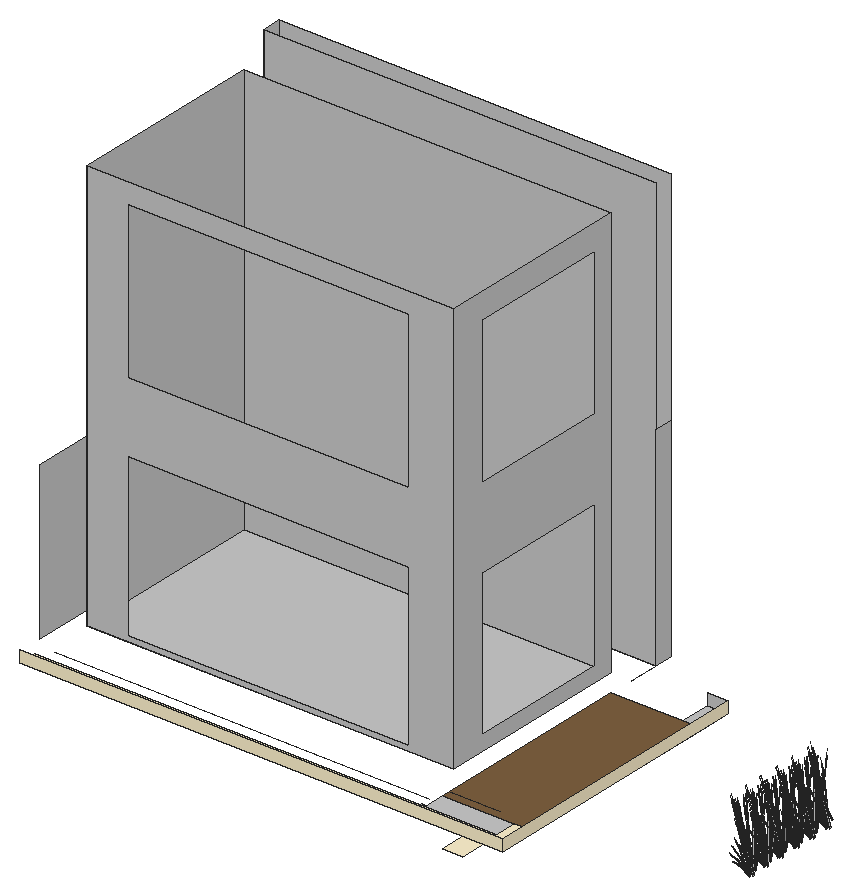
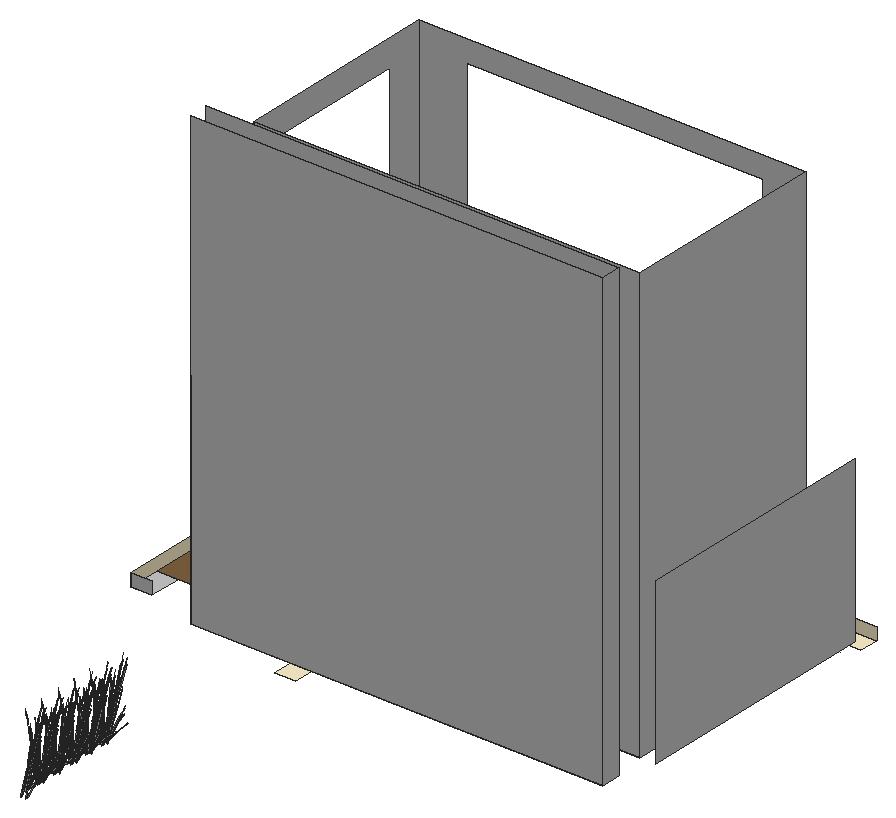
# SketchUp Ruby script. Lengths in inches.
U = 1.inch
M = Sketchup.active_model
def pt(a) = Geom::Point3d.new(a.map { |v| v * U })
def face(e, loops, mat)
  f = e.add_face(loops[0].map { |a| pt(a) })
  loops[1..].each { |l| e.add_face(l.map { |a| pt(a) }).erase! }
  f.material = f.back_material = mat if mat
  f
end
# faces: each face lists its corners as indices into pts; further lists are holes
def faces(e, pts, list, mat = nil) = list.each { |f| face(e, (f[0].is_a?(Array) ? f : [f]).map { |l| l.map { |i| pts[i] } }, mat) }
# xy, xz, yz: faces in a plane at the given z, y or x. An outline is a flat list of corners, or four numbers for a rectangle; further outlines are holes
def ring(l) = l.size == 4 ? [[l[0], l[1]], [l[2], l[1]], [l[2], l[3]], [l[0], l[3]]] : l.each_slice(2).to_a
def flat(e, list, mat, &to3) = list.each { |f| face(e, (f[0].is_a?(Array) ? f : [f]).map { |l| ring(l).map { |u, v| to3.(u, v) } }, mat) }
def xy(e, z, list, mat = nil) = flat(e, list, mat) { |x, y| [x, y, z] }
def xz(e, y, list, mat = nil) = flat(e, list, mat) { |x, z| [x, y, z] }
def yz(e, x, list, mat = nil) = flat(e, list, mat) { |y, z| [x, y, z] }
def lines(e, pts, list) = list.each { |a, b| e.add_line(pt(pts[a]), pt(pts[b])) }
# prism: a flat outline (further loops are holes) pulled along v
def prism(e, loops, v, mat = nil)
  f = face(e, loops, mat); d = Geom::Vector3d.new(v.map { |x| x * U })
  f.pushpull(f.normal.samedirection?(d) ? d.length : -d.length)
end
def box(e, o, s, mat = nil) = prism(e, [[o, [o[0] + s[0], o[1], o[2]], [o[0] + s[0], o[1] + s[1], o[2]], [o[0], o[1] + s[1], o[2]]]], [0, 0, s[2]], mat)
def at(x, y, z, deg = 0) = Geom::Transformation.translation(pt([x, y, z])) * Geom::Transformation.rotation(ORIGIN, Z_AXIS, deg.degrees)
def axes(o, x, y, z) = Geom::Transformation.new([*x, 0, *y, 0, *z, 0, *pt(o).to_a, 1])
def part(name) = M.definitions.add(name)
# library, detail: a bought-in or finely detailed component or shape, given as its bounding box
def library(name, o, s) = part(name).tap { |d| box(d.entities, o, s) }
def detail(e, o, s) = box(e.add_group.entities, o, s)
def put(e, d, t, mat = nil) = e.add_instance(d, t).tap { |i| i.material = mat if mat }
def group(e, t, mat = nil) = e.add_group.tap { |g| g.transformation = t; g.material = mat if mat }.entities
root = M.entities
M.materials.add("D01_Frost_White").color = [255, 242, 206]
M.materials.add("LightPink_Translucent").color = [144, 107, 117]
M.materials["LightPink_Translucent"].alpha = 0.75
M.materials.add("Plywood_01_1K").color = [125, 96, 64]
M.materials.add("[_0053_Ivory_]").color = [200, 200, 200]
c1 = part("blade")
p = [[2.15,0.21,22],[0,0.17,0],[0.09,0.45,0],[2.18,0.31,22],[2.29,0.31,22],[0.38,0.45,0],
  [2.48,0.24,33],[2.49,0.24,33],[2.48,0.22,33]]
faces(c1.entities,p,[[0,1,2,3],[4,5,2,3],[6,3,4,7],[8,0,3,6]])
c2 = part("seeds")
p = [[0.3,-0.1,1.38],[-0.01,-0.03,1.59],[-0.01,-0.03,0.03],[0.14,-0.07,-0.07],[0.29,-0.03,3],[0.15,0.01,3.11]]
faces(c2.entities,p,[[0,1,2,3],[1,0,4,5]],"LightPink_Translucent")
c3 = part("blade with seeds")
put(c3.entities,c1,at(0,0,0))
put(c3.entities,c2,axes([2.4,0.25,30.99],[1.5799,-0.05474,1.17369],[-0.12525,1.92788,0.29478],[-0.07173,-0.02425,1.56792]))
xy(root,81,[[598.7,122.15,610.51,146.15],[598.51,149.15,610.51,170.15],[598.51,173.15,610.51,194.15],[598.51,197.15,610.51,218.15]],"D01_Frost_White")
xy(root,120,[[377.51,83.15,377.51,94.15,653.51,94.15,653.51,107.15,665.51,107.15,665.51,83.15]],"D01_Frost_White")
xy(root,120,[[610.51,107.15,665.51,233.15]],"Plywood_01_1K")
xy(root,120,[[607.51,94.15,607.51,95.51,610.51,95.51,610.51,107.15,653.51,107.15,653.51,94.15],[653.51,233.15,665.51,251.15]],"[_0053_Ivory_]")
xy(root,126,[[386.51,122.15,605.51,239.15],[383.51,257.92,617.51,269.15]],"[_0053_Ivory_]")
xz(root,83.15,[[377.51,120,665.51,127]],"D01_Frost_White")
xz(root,122.15,[[[386.51,126,605.51,372],[410.51,129,578.51,225],[410.51,267,578.51,360]]],"[_0053_Ivory_]")
xz(root,239.15,[[386.51,126,605.51,372]],"[_0053_Ivory_]")
xz(root,251.15,[[653.51,120,665.51,127]],"[_0053_Ivory_]")
xz(root,257.92,[[383.51,126,617.51,384]],"[_0053_Ivory_]")
xz(root,269.15,[[383.51,126,617.51,384]],"[_0053_Ivory_]")
yz(root,377.51,[[98.15,126,239.15,219]],"[_0053_Ivory_]")
yz(root,383.51,[[257.92,126,269.15,384]],"[_0053_Ivory_]")
yz(root,386.51,[[122.15,126,239.15,372]],"[_0053_Ivory_]")
yz(root,605.51,[[[122.15,126,239.15,372],[143.15,270,227.15,357],[143.15,135,227.15,222]]],"[_0053_Ivory_]")
yz(root,617.51,[[257.92,126,269.15,252]],"[_0053_Ivory_]")
yz(root,665.51,[[83.15,120,251.15,127]],"D01_Frost_White")
p = [[617.51,239.15,126],[617.51,257.92,126],[607.51,101.15,120],[383.51,101.15,120],[617.51,104.15,126],[647.51,104.15,126]]
lines(root,p,[[0,1],[2,3],[4,5]])
put(root,c3,axes([672.63,315.29,38.36],[-0.01133,0.07538,1.77383],[-0.55883,0.27355,-0.16761],[-0.16445,-0.13983,0.31391]),"[_0053_Ivory_]")
put(root,c3,axes([672.51,316.63,38.75],[0.67657,-0.16163,0.53763],[0.11742,0.63404,0.4433],[-0.15912,-0.18687,1.11249]),"[_0053_Ivory_]")
put(root,c3,axes([673.27,315.58,38.37],[-0.0929,-0.08817,1.74944],[-0.61994,0.0559,-0.27667],[-0.09894,-0.21089,0.14031]),"[_0053_Ivory_]")
put(root,c3,axes([676.54,254.36,38.37],[-0.09918,0.08165,1.74944],[0.00844,0.59653,-0.27667],[-0.22734,0.07758,0.14031]),"[_0053_Ivory_]")
put(root,c3,axes([676.54,265.51,38.37],[-0.09918,0.08165,1.74944],[0.00844,0.59653,-0.27667],[-0.22734,0.07758,0.14031]),"[_0053_Ivory_]")
put(root,c3,axes([676.54,276.5,38.37],[-0.09918,0.08165,1.74944],[0.00844,0.59653,-0.27667],[-0.22734,0.07758,0.14031]),"[_0053_Ivory_]")
put(root,c3,axes([676.54,288.54,38.37],[-0.09918,0.08165,1.74944],[0.00844,0.59653,-0.27667],[-0.22734,0.07758,0.14031]),"[_0053_Ivory_]")
put(root,c3,axes([676.54,299.91,38.37],[-0.09918,0.08165,1.74944],[0.00844,0.59653,-0.27667],[-0.22734,0.07758,0.14031]),"[_0053_Ivory_]")
put(root,c3,axes([675.4375,254.96,38.36],[0.07751,0.01687,1.77383],[0.23978,0.55562,-0.16761],[-0.15867,0.14583,0.31391]),"[_0053_Ivory_]")
put(root,c3,axes([675.4375,266.11,38.36],[0.07751,0.01687,1.77383],[0.23978,0.55562,-0.16761],[-0.15867,0.14583,0.31391]),"[_0053_Ivory_]")
put(root,c3,axes([675.4375,277.1,38.36],[0.07751,0.01687,1.77383],[0.23978,0.55562,-0.16761],[-0.15867,0.14583,0.31391]),"[_0053_Ivory_]")
put(root,c3,axes([675.4375,289.14,38.36],[0.07751,0.01687,1.77383],[0.23978,0.55562,-0.16761],[-0.15867,0.14583,0.31391]),"[_0053_Ivory_]")
put(root,c3,axes([675.4375,300.51,38.36],[0.07751,0.01687,1.77383],[0.23978,0.55562,-0.16761],[-0.15867,0.14583,0.31391]),"[_0053_Ivory_]")
put(root,c3,axes([677.01,251.875,38.36],[0.04503,0.06276,1.77383],[-0.21706,0.56413,-0.16761],[-0.21983,0.00408,0.31391]),"[_0053_Ivory_]")
put(root,c3,axes([677.01,263.02,38.36],[0.04503,0.06276,1.77383],[-0.21706,0.56413,-0.16761],[-0.21983,0.00408,0.31391]),"[_0053_Ivory_]")
put(root,c3,axes([677.01,274.01,38.36],[0.04503,0.06276,1.77383],[-0.21706,0.56413,-0.16761],[-0.21983,0.00408,0.31391]),"[_0053_Ivory_]")
put(root,c3,axes([677.01,286.06,38.36],[0.04503,0.06276,1.77383],[-0.21706,0.56413,-0.16761],[-0.21983,0.00408,0.31391]),"[_0053_Ivory_]")
put(root,c3,axes([677.01,297.43,38.36],[0.04503,0.06276,1.77383],[-0.21706,0.56413,-0.16761],[-0.21983,0.00408,0.31391]),"[_0053_Ivory_]")
put(root,c3,axes([677.01,309.4,38.36],[0.04503,0.06276,1.77383],[-0.21706,0.56413,-0.16761],[-0.21983,0.00408,0.31391]),"[_0053_Ivory_]")
put(root,c3,axes([677.51,251.5,38.37],[-0.13068,-0.00444,1.74944],[-0.41604,0.44388,-0.27667],[-0.22198,-0.0907,0.14031]),"[_0053_Ivory_]")
put(root,c3,axes([677.51,262.65,38.37],[-0.13068,-0.00444,1.74944],[-0.41604,0.44388,-0.27667],[-0.22198,-0.0907,0.14031]),"[_0053_Ivory_]")
put(root,c3,axes([677.51,273.64,38.37],[-0.13068,-0.00444,1.74944],[-0.41604,0.44388,-0.27667],[-0.22198,-0.0907,0.14031]),"[_0053_Ivory_]")
put(root,c3,axes([677.51,285.68,38.37],[-0.13068,-0.00444,1.74944],[-0.41604,0.44388,-0.27667],[-0.22198,-0.0907,0.14031]),"[_0053_Ivory_]")
put(root,c3,axes([677.51,297.05,38.37],[-0.13068,-0.00444,1.74944],[-0.41604,0.44388,-0.27667],[-0.22198,-0.0907,0.14031]),"[_0053_Ivory_]")
put(root,c3,axes([677.51,309.03,38.37],[-0.13068,-0.00444,1.74944],[-0.41604,0.44388,-0.27667],[-0.22198,-0.0907,0.14031]),"[_0053_Ivory_]")
put(root,c3,axes([676.98,253.95,38.39],[0.17159,-0.57338,0.48003],[0.56413,0.19607,0.3958],[-0.22185,0.03446,0.9933]),"[_0053_Ivory_]")
put(root,c3,axes([676.98,265.1,38.39],[0.17159,-0.57338,0.48003],[0.56413,0.19607,0.3958],[-0.22185,0.03446,0.9933]),"[_0053_Ivory_]")
put(root,c3,axes([676.98,276.09,38.39],[0.17159,-0.57338,0.48003],[0.56413,0.19607,0.3958],[-0.22185,0.03446,0.9933]),"[_0053_Ivory_]")
put(root,c3,axes([676.98,288.14,38.39],[0.17159,-0.57338,0.48003],[0.56413,0.19607,0.3958],[-0.22185,0.03446,0.9933]),"[_0053_Ivory_]")
put(root,c3,axes([676.98,299.5,38.39],[0.17159,-0.57338,0.48003],[0.56413,0.19607,0.3958],[-0.22185,0.03446,0.9933]),"[_0053_Ivory_]")
put(root,c3,axes([676.98,311.48,38.39],[0.17159,-0.57338,0.48003],[0.56413,0.19607,0.3958],[-0.22185,0.03446,0.9933]),"[_0053_Ivory_]")
put(root,c3,axes([677.18,253.79,38.6875],[0.30559,0.56943,-0.1216],[-0.54237,0.27983,-0.67495],[-0.22856,0.07513,1.02557]),"[_0053_Ivory_]")
put(root,c3,axes([677.18,264.9375,38.6875],[0.30559,0.56943,-0.1216],[-0.54237,0.27983,-0.67495],[-0.22856,0.07513,1.02557]),"[_0053_Ivory_]")
put(root,c3,axes([677.18,275.93,38.6875],[0.30559,0.56943,-0.1216],[-0.54237,0.27983,-0.67495],[-0.22856,0.07513,1.02557]),"[_0053_Ivory_]")
put(root,c3,axes([677.18,287.97,38.6875],[0.30559,0.56943,-0.1216],[-0.54237,0.27983,-0.67495],[-0.22856,0.07513,1.02557]),"[_0053_Ivory_]")
put(root,c3,axes([677.18,299.34,38.6875],[0.30559,0.56943,-0.1216],[-0.54237,0.27983,-0.67495],[-0.22856,0.07513,1.02557]),"[_0053_Ivory_]")
put(root,c3,axes([677.87,252.61,38.6875],[-0.03252,0.63953,-0.1216],[-0.61574,-0.01748,-0.67495],[-0.23714,-0.04442,1.02557]),"[_0053_Ivory_]")
put(root,c3,axes([677.87,263.75,38.6875],[-0.03252,0.63953,-0.1216],[-0.61574,-0.01748,-0.67495],[-0.23714,-0.04442,1.02557]),"[_0053_Ivory_]")
put(root,c3,axes([677.87,274.75,38.6875],[-0.03252,0.63953,-0.1216],[-0.61574,-0.01748,-0.67495],[-0.23714,-0.04442,1.02557]),"[_0053_Ivory_]")
put(root,c3,axes([677.87,286.79,38.6875],[-0.03252,0.63953,-0.1216],[-0.61574,-0.01748,-0.67495],[-0.23714,-0.04442,1.02557]),"[_0053_Ivory_]")
put(root,c3,axes([677.87,298.16,38.6875],[-0.03252,0.63953,-0.1216],[-0.61574,-0.01748,-0.67495],[-0.23714,-0.04442,1.02557]),"[_0053_Ivory_]")
put(root,c3,axes([677.87,310.13,38.6875],[-0.03252,0.63953,-0.1216],[-0.61574,-0.01748,-0.67495],[-0.23714,-0.04442,1.02557]),"[_0053_Ivory_]")
put(root,c3,axes([676.93,253.8,38.38],[-0.22307,-0.42878,0.0643],[0.40677,-0.20987,0.50621],[-0.17931,0.04141,0.77189]),"[_0053_Ivory_]")
put(root,c3,axes([676.93,264.95,38.38],[-0.22307,-0.42878,0.0643],[0.40677,-0.20987,0.50621],[-0.17931,0.04141,0.77189]),"[_0053_Ivory_]")
put(root,c3,axes([676.93,275.94,38.38],[-0.22307,-0.42878,0.0643],[0.40677,-0.20987,0.50621],[-0.17931,0.04141,0.77189]),"[_0053_Ivory_]")
put(root,c3,axes([676.93,287.98,38.38],[-0.22307,-0.42878,0.0643],[0.40677,-0.20987,0.50621],[-0.17931,0.04141,0.77189]),"[_0053_Ivory_]")
put(root,c3,axes([676.93,299.35,38.38],[-0.22307,-0.42878,0.0643],[0.40677,-0.20987,0.50621],[-0.17931,0.04141,0.77189]),"[_0053_Ivory_]")
put(root,c3,axes([676.93,311.33,38.38],[-0.22307,-0.42878,0.0643],[0.40677,-0.20987,0.50621],[-0.17931,0.04141,0.77189]),"[_0053_Ivory_]")
put(root,c3,axes([677.11,255.38,38.39],[-0.15063,-0.57876,0.48003],[0.59087,-0.10045,0.3958],[-0.17414,0.13612,0.9933]),"[_0053_Ivory_]")
put(root,c3,axes([677.11,266.53,38.39],[-0.15063,-0.57876,0.48003],[0.59087,-0.10045,0.3958],[-0.17414,0.13612,0.9933]),"[_0053_Ivory_]")
put(root,c3,axes([677.11,277.52,38.39],[-0.15063,-0.57876,0.48003],[0.59087,-0.10045,0.3958],[-0.17414,0.13612,0.9933]),"[_0053_Ivory_]")
put(root,c3,axes([677.11,289.56,38.39],[-0.15063,-0.57876,0.48003],[0.59087,-0.10045,0.3958],[-0.17414,0.13612,0.9933]),"[_0053_Ivory_]")
put(root,c3,axes([677.11,300.93,38.39],[-0.15063,-0.57876,0.48003],[0.59087,-0.10045,0.3958],[-0.17414,0.13612,0.9933]),"[_0053_Ivory_]")
put(root,c3,axes([677.42,252.5,38.75],[0.50157,-0.46409,0.53763],[0.43258,0.49285,0.4433],[-0.23532,-0.08561,1.11249]),"[_0053_Ivory_]")
put(root,c3,axes([677.42,263.65,38.75],[0.50157,-0.46409,0.53763],[0.43258,0.49285,0.4433],[-0.23532,-0.08561,1.11249]),"[_0053_Ivory_]")
put(root,c3,axes([677.42,274.64,38.75],[0.50157,-0.46409,0.53763],[0.43258,0.49285,0.4433],[-0.23532,-0.08561,1.11249]),"[_0053_Ivory_]")
put(root,c3,axes([677.42,286.6875,38.75],[0.50157,-0.46409,0.53763],[0.43258,0.49285,0.4433],[-0.23532,-0.08561,1.11249]),"[_0053_Ivory_]")
put(root,c3,axes([677.42,298.05,38.75],[0.50157,-0.46409,0.53763],[0.43258,0.49285,0.4433],[-0.23532,-0.08561,1.11249]),"[_0053_Ivory_]")
put(root,c3,axes([677.42,310.03,38.75],[0.50157,-0.46409,0.53763],[0.43258,0.49285,0.4433],[-0.23532,-0.08561,1.11249]),"[_0053_Ivory_]")
put(root,c3,axes([677,255.27,38.38],[-0.41695,-0.26447,0.0643],[0.24275,-0.37662,0.50621],[-0.13368,0.12176,0.77189]),"[_0053_Ivory_]")
put(root,c3,axes([677,266.42,38.38],[-0.41695,-0.26447,0.0643],[0.24275,-0.37662,0.50621],[-0.13368,0.12176,0.77189]),"[_0053_Ivory_]")
put(root,c3,axes([677,277.41,38.38],[-0.41695,-0.26447,0.0643],[0.24275,-0.37662,0.50621],[-0.13368,0.12176,0.77189]),"[_0053_Ivory_]")
put(root,c3,axes([677,289.45,38.38],[-0.41695,-0.26447,0.0643],[0.24275,-0.37662,0.50621],[-0.13368,0.12176,0.77189]),"[_0053_Ivory_]")
put(root,c3,axes([677,300.82,38.38],[-0.41695,-0.26447,0.0643],[0.24275,-0.37662,0.50621],[-0.13368,0.12176,0.77189]),"[_0053_Ivory_]")
put(root,c3,axes([677.39,253.96,38.7],[0.50475,0.17543,0.35414],[-0.14722,0.5118,-0.4572],[-0.20322,0.04693,0.87481]),"[_0053_Ivory_]")
put(root,c3,axes([677.39,265.11,38.7],[0.50475,0.17543,0.35414],[-0.14722,0.5118,-0.4572],[-0.20322,0.04693,0.87481]),"[_0053_Ivory_]")
put(root,c3,axes([677.39,276.1,38.7],[0.50475,0.17543,0.35414],[-0.14722,0.5118,-0.4572],[-0.20322,0.04693,0.87481]),"[_0053_Ivory_]")
put(root,c3,axes([677.39,288.14,38.7],[0.50475,0.17543,0.35414],[-0.14722,0.5118,-0.4572],[-0.20322,0.04693,0.87481]),"[_0053_Ivory_]")
put(root,c3,axes([677.39,299.51,38.7],[0.50475,0.17543,0.35414],[-0.14722,0.5118,-0.4572],[-0.20322,0.04693,0.87481]),"[_0053_Ivory_]")
put(root,c3,axes([677.39,311.49,38.7],[0.50475,0.17543,0.35414],[-0.14722,0.5118,-0.4572],[-0.20322,0.04693,0.87481]),"[_0053_Ivory_]")
put(root,c3,axes([677.65,252.5,38.38],[0.03058,-0.47819,0.0643],[0.4618,0.01311,0.50621],[-0.1769,-0.05004,0.77189]),"[_0053_Ivory_]")
put(root,c3,axes([677.65,263.65,38.38],[0.03058,-0.47819,0.0643],[0.4618,0.01311,0.50621],[-0.1769,-0.05004,0.77189]),"[_0053_Ivory_]")
put(root,c3,axes([677.65,274.64,38.38],[0.03058,-0.47819,0.0643],[0.4618,0.01311,0.50621],[-0.1769,-0.05004,0.77189]),"[_0053_Ivory_]")
put(root,c3,axes([677.65,286.68,38.38],[0.03058,-0.47819,0.0643],[0.4618,0.01311,0.50621],[-0.1769,-0.05004,0.77189]),"[_0053_Ivory_]")
put(root,c3,axes([677.65,298.05,38.38],[0.03058,-0.47819,0.0643],[0.4618,0.01311,0.50621],[-0.1769,-0.05004,0.77189]),"[_0053_Ivory_]")
put(root,c3,axes([677.65,310.03,38.38],[0.03058,-0.47819,0.0643],[0.4618,0.01311,0.50621],[-0.1769,-0.05004,0.77189]),"[_0053_Ivory_]")
put(root,c3,axes([676.56,256.58,38.37],[-0.0151,0.12444,1.74944],[0.42844,0.43292,-0.27667],[-0.11216,0.20472,0.14031]),"[_0053_Ivory_]")
put(root,c3,axes([676.56,267.73,38.37],[-0.0151,0.12444,1.74944],[0.42844,0.43292,-0.27667],[-0.11216,0.20472,0.14031]),"[_0053_Ivory_]")
put(root,c3,axes([676.56,278.72,38.37],[-0.0151,0.12444,1.74944],[0.42844,0.43292,-0.27667],[-0.11216,0.20472,0.14031]),"[_0053_Ivory_]")
put(root,c3,axes([676.56,290.77,38.37],[-0.0151,0.12444,1.74944],[0.42844,0.43292,-0.27667],[-0.11216,0.20472,0.14031]),"[_0053_Ivory_]")
put(root,c3,axes([676.56,302.14,38.37],[-0.0151,0.12444,1.74944],[0.42844,0.43292,-0.27667],[-0.11216,0.20472,0.14031]),"[_0053_Ivory_]")
put(root,c3,axes([679.07,251.67,39.08],[-0.40534,0.60286,-0.13619],[-0.58702,-0.34732,-0.75594],[-0.20405,-0.17032,1.14864]),"[_0053_Ivory_]")
put(root,c3,axes([679.07,262.82,39.08],[-0.40534,0.60286,-0.13619],[-0.58702,-0.34732,-0.75594],[-0.20405,-0.17032,1.14864]),"[_0053_Ivory_]")
put(root,c3,axes([679.07,273.8125,39.08],[-0.40534,0.60286,-0.13619],[-0.58702,-0.34732,-0.75594],[-0.20405,-0.17032,1.14864]),"[_0053_Ivory_]")
put(root,c3,axes([679.07,285.85,39.08],[-0.40534,0.60286,-0.13619],[-0.58702,-0.34732,-0.75594],[-0.20405,-0.17032,1.14864]),"[_0053_Ivory_]")
put(root,c3,axes([679.07,297.22,39.08],[-0.40534,0.60286,-0.13619],[-0.58702,-0.34732,-0.75594],[-0.20405,-0.17032,1.14864]),"[_0053_Ivory_]")
put(root,c3,axes([679.07,309.2,39.08],[-0.40534,0.60286,-0.13619],[-0.58702,-0.34732,-0.75594],[-0.20405,-0.17032,1.14864]),"[_0053_Ivory_]")
put(root,c3,axes([677.96,252.86,38.7],[0.34557,0.39372,0.35414],[-0.39459,0.37271,-0.4572],[-0.20048,-0.05671,0.87481]),"[_0053_Ivory_]")
put(root,c3,axes([677.96,264.01,38.7],[0.34557,0.39372,0.35414],[-0.39459,0.37271,-0.4572],[-0.20048,-0.05671,0.87481]),"[_0053_Ivory_]")
put(root,c3,axes([677.96,275,38.7],[0.34557,0.39372,0.35414],[-0.39459,0.37271,-0.4572],[-0.20048,-0.05671,0.87481]),"[_0053_Ivory_]")
put(root,c3,axes([677.96,287.04,38.7],[0.34557,0.39372,0.35414],[-0.39459,0.37271,-0.4572],[-0.20048,-0.05671,0.87481]),"[_0053_Ivory_]")
put(root,c3,axes([677.96,298.41,38.7],[0.34557,0.39372,0.35414],[-0.39459,0.37271,-0.4572],[-0.20048,-0.05671,0.87481]),"[_0053_Ivory_]")
put(root,c3,axes([677.96,310.38,38.7],[0.34557,0.39372,0.35414],[-0.39459,0.37271,-0.4572],[-0.20048,-0.05671,0.87481]),"[_0053_Ivory_]")
put(root,c3,axes([677.2,255.14,38.6875],[0.56181,0.34675,-0.1216],[-0.32367,0.50216,-0.67495],[-0.15873,0.17455,1.02557]),"[_0053_Ivory_]")
put(root,c3,axes([677.2,266.29,38.6875],[0.56181,0.34675,-0.1216],[-0.32367,0.50216,-0.67495],[-0.15873,0.17455,1.02557]),"[_0053_Ivory_]")
put(root,c3,axes([677.2,277.28,38.6875],[0.56181,0.34675,-0.1216],[-0.32367,0.50216,-0.67495],[-0.15873,0.17455,1.02557]),"[_0053_Ivory_]")
put(root,c3,axes([677.2,289.33,38.6875],[0.56181,0.34675,-0.1216],[-0.32367,0.50216,-0.67495],[-0.15873,0.17455,1.02557]),"[_0053_Ivory_]")
put(root,c3,axes([677.2,300.69,38.6875],[0.56181,0.34675,-0.1216],[-0.32367,0.50216,-0.67495],[-0.15873,0.17455,1.02557]),"[_0053_Ivory_]")
put(root,c3,axes([675.92,316.21,38.36],[-0.06168,0.04803,1.77383],[-0.60432,-0.16205,-0.16761],[-0.02188,-0.20961,0.31391]),"[_0053_Ivory_]")
put(root,c3,axes([676.28,256.65,39.3],[0.53595,0.16786,-0.06488],[-0.16486,0.51664,-0.29416],[-0.08766,0.07844,0.97024]),"[_0053_Ivory_]")
put(root,c3,axes([676.28,267.8,39.3],[0.53595,0.16786,-0.06488],[-0.16486,0.51664,-0.29416],[-0.08766,0.07844,0.97024]),"[_0053_Ivory_]")
put(root,c3,axes([676.28,278.79,39.3],[0.53595,0.16786,-0.06488],[-0.16486,0.51664,-0.29416],[-0.08766,0.07844,0.97024]),"[_0053_Ivory_]")
put(root,c3,axes([676.28,290.83,39.3],[0.53595,0.16786,-0.06488],[-0.16486,0.51664,-0.29416],[-0.08766,0.07844,0.97024]),"[_0053_Ivory_]")
put(root,c3,axes([676.28,302.2,39.3],[0.53595,0.16786,-0.06488],[-0.16486,0.51664,-0.29416],[-0.08766,0.07844,0.97024]),"[_0053_Ivory_]")
put(root,c3,axes([677.48,255.1875,38.7],[0.52868,-0.08987,0.35414],[0.1396,0.51376,-0.4572],[-0.1515,0.13799,0.87481]),"[_0053_Ivory_]")
put(root,c3,axes([677.48,266.34,38.7],[0.52868,-0.08987,0.35414],[0.1396,0.51376,-0.4572],[-0.1515,0.13799,0.87481]),"[_0053_Ivory_]")
put(root,c3,axes([677.48,277.33,38.7],[0.52868,-0.08987,0.35414],[0.1396,0.51376,-0.4572],[-0.1515,0.13799,0.87481]),"[_0053_Ivory_]")
put(root,c3,axes([677.48,289.37,38.7],[0.52868,-0.08987,0.35414],[0.1396,0.51376,-0.4572],[-0.1515,0.13799,0.87481]),"[_0053_Ivory_]")
put(root,c3,axes([677.48,300.74,38.7],[0.52868,-0.08987,0.35414],[0.1396,0.51376,-0.4572],[-0.1515,0.13799,0.87481]),"[_0053_Ivory_]")
put(root,c3,axes([678.91,250.24,38.36],[-0.01133,0.07538,1.77383],[-0.55883,0.27355,-0.16761],[-0.16445,-0.13983,0.31391]),"[_0053_Ivory_]")
put(root,c3,axes([678.91,261.39,38.36],[-0.01133,0.07538,1.77383],[-0.55883,0.27355,-0.16761],[-0.16445,-0.13983,0.31391]),"[_0053_Ivory_]")
put(root,c3,axes([678.91,272.38,38.36],[-0.01133,0.07538,1.77383],[-0.55883,0.27355,-0.16761],[-0.16445,-0.13983,0.31391]),"[_0053_Ivory_]")
put(root,c3,axes([678.91,284.42,38.36],[-0.01133,0.07538,1.77383],[-0.55883,0.27355,-0.16761],[-0.16445,-0.13983,0.31391]),"[_0053_Ivory_]")
put(root,c3,axes([678.91,295.79,38.36],[-0.01133,0.07538,1.77383],[-0.55883,0.27355,-0.16761],[-0.16445,-0.13983,0.31391]),"[_0053_Ivory_]")
put(root,c3,axes([678.91,307.77,38.36],[-0.01133,0.07538,1.77383],[-0.55883,0.27355,-0.16761],[-0.16445,-0.13983,0.31391]),"[_0053_Ivory_]")
put(root,c3,axes([677.98,256.55,38.39],[-0.43249,-0.42907,0.48003],[0.45929,-0.37004,0.3958],[-0.07978,0.2013,0.9933]),"[_0053_Ivory_]")
put(root,c3,axes([677.98,267.7,38.39],[-0.43249,-0.42907,0.48003],[0.45929,-0.37004,0.3958],[-0.07978,0.2013,0.9933]),"[_0053_Ivory_]")
put(root,c3,axes([677.98,278.69,38.39],[-0.43249,-0.42907,0.48003],[0.45929,-0.37004,0.3958],[-0.07978,0.2013,0.9933]),"[_0053_Ivory_]")
put(root,c3,axes([677.98,290.74,38.39],[-0.43249,-0.42907,0.48003],[0.45929,-0.37004,0.3958],[-0.07978,0.2013,0.9933]),"[_0053_Ivory_]")
put(root,c3,axes([677.98,302.1,38.39],[-0.43249,-0.42907,0.48003],[0.45929,-0.37004,0.3958],[-0.07978,0.2013,0.9933]),"[_0053_Ivory_]")
put(root,c3,axes([677.82,256.51,38.38],[-0.49911,-0.0293,0.0643],[0.01368,-0.44245,0.50621],[-0.05223,0.16948,0.77189]),"[_0053_Ivory_]")
put(root,c3,axes([677.82,267.66,38.38],[-0.49911,-0.0293,0.0643],[0.01368,-0.44245,0.50621],[-0.05223,0.16948,0.77189]),"[_0053_Ivory_]")
put(root,c3,axes([677.82,278.65,38.38],[-0.49911,-0.0293,0.0643],[0.01368,-0.44245,0.50621],[-0.05223,0.16948,0.77189]),"[_0053_Ivory_]")
put(root,c3,axes([677.82,290.7,38.38],[-0.49911,-0.0293,0.0643],[0.01368,-0.44245,0.50621],[-0.05223,0.16948,0.77189]),"[_0053_Ivory_]")
put(root,c3,axes([677.82,302.0625,38.38],[-0.49911,-0.0293,0.0643],[0.01368,-0.44245,0.50621],[-0.05223,0.16948,0.77189]),"[_0053_Ivory_]")
put(root,c3,axes([679.03,252.17,38.7],[0.0938,0.50652,0.35414],[-0.53623,0.13375,-0.4572],[-0.14403,-0.14515,0.87481]),"[_0053_Ivory_]")
put(root,c3,axes([679.03,263.32,38.7],[0.0938,0.50652,0.35414],[-0.53623,0.13375,-0.4572],[-0.14403,-0.14515,0.87481]),"[_0053_Ivory_]")
put(root,c3,axes([679.03,274.3125,38.7],[0.0938,0.50652,0.35414],[-0.53623,0.13375,-0.4572],[-0.14403,-0.14515,0.87481]),"[_0053_Ivory_]")
put(root,c3,axes([679.03,286.36,38.7],[0.0938,0.50652,0.35414],[-0.53623,0.13375,-0.4572],[-0.14403,-0.14515,0.87481]),"[_0053_Ivory_]")
put(root,c3,axes([679.03,297.72,38.7],[0.0938,0.50652,0.35414],[-0.53623,0.13375,-0.4572],[-0.14403,-0.14515,0.87481]),"[_0053_Ivory_]")
put(root,c3,axes([679.03,309.7,38.7],[0.0938,0.50652,0.35414],[-0.53623,0.13375,-0.4572],[-0.14403,-0.14515,0.87481]),"[_0053_Ivory_]")
put(root,c3,axes([676.51,257.86,38.36],[0.0689,-0.03797,1.77383],[0.5695,0.25254,-0.16761],[-0.01338,0.21027,0.31391]),"[_0053_Ivory_]")
put(root,c3,axes([676.51,269.01,38.36],[0.0689,-0.03797,1.77383],[0.5695,0.25254,-0.16761],[-0.01338,0.21027,0.31391]),"[_0053_Ivory_]")
put(root,c3,axes([676.51,280,38.36],[0.0689,-0.03797,1.77383],[0.5695,0.25254,-0.16761],[-0.01338,0.21027,0.31391]),"[_0053_Ivory_]")
put(root,c3,axes([676.51,292.04,38.36],[0.0689,-0.03797,1.77383],[0.5695,0.25254,-0.16761],[-0.01338,0.21027,0.31391]),"[_0053_Ivory_]")
put(root,c3,axes([676.51,303.41,38.36],[0.0689,-0.03797,1.77383],[0.5695,0.25254,-0.16761],[-0.01338,0.21027,0.31391]),"[_0053_Ivory_]")
put(root,c3,axes([678.79,251.58,38.75],[0.67657,-0.16163,0.53763],[0.11742,0.63404,0.4433],[-0.15912,-0.18687,1.11249]),"[_0053_Ivory_]")
put(root,c3,axes([678.79,262.73,38.75],[0.67657,-0.16163,0.53763],[0.11742,0.63404,0.4433],[-0.15912,-0.18687,1.11249]),"[_0053_Ivory_]")
put(root,c3,axes([678.79,273.72,38.75],[0.67657,-0.16163,0.53763],[0.11742,0.63404,0.4433],[-0.15912,-0.18687,1.11249]),"[_0053_Ivory_]")
put(root,c3,axes([678.79,285.76,38.75],[0.67657,-0.16163,0.53763],[0.11742,0.63404,0.4433],[-0.15912,-0.18687,1.11249]),"[_0053_Ivory_]")
put(root,c3,axes([678.79,297.13,38.75],[0.67657,-0.16163,0.53763],[0.11742,0.63404,0.4433],[-0.15912,-0.18687,1.11249]),"[_0053_Ivory_]")
put(root,c3,axes([678.79,309.1,38.75],[0.67657,-0.16163,0.53763],[0.11742,0.63404,0.4433],[-0.15912,-0.18687,1.11249]),"[_0053_Ivory_]")
put(root,c3,axes([678.94,251.71,38.38],[0.27604,-0.39948,0.0643],[0.39309,0.23258,0.50621],[-0.12709,-0.12808,0.77189]),"[_0053_Ivory_]")
put(root,c3,axes([678.94,262.86,38.38],[0.27604,-0.39948,0.0643],[0.39309,0.23258,0.50621],[-0.12709,-0.12808,0.77189]),"[_0053_Ivory_]")
put(root,c3,axes([678.94,273.85,38.38],[0.27604,-0.39948,0.0643],[0.39309,0.23258,0.50621],[-0.12709,-0.12808,0.77189]),"[_0053_Ivory_]")
put(root,c3,axes([678.94,285.9,38.38],[0.27604,-0.39948,0.0643],[0.39309,0.23258,0.50621],[-0.12709,-0.12808,0.77189]),"[_0053_Ivory_]")
put(root,c3,axes([678.94,297.26,38.38],[0.27604,-0.39948,0.0643],[0.39309,0.23258,0.50621],[-0.12709,-0.12808,0.77189]),"[_0053_Ivory_]")
put(root,c3,axes([678.94,309.24,38.38],[0.27604,-0.39948,0.0643],[0.39309,0.23258,0.50621],[-0.12709,-0.12808,0.77189]),"[_0053_Ivory_]")
put(root,c3,axes([676.05,316.66,38.37],[-0.00586,-0.12516,1.74944],[-0.49517,-0.36172,-0.27667],[0.07656,-0.21927,0.14031]),"[_0053_Ivory_]")
put(root,c3,axes([679.55,250.53,38.37],[-0.0929,-0.08817,1.74944],[-0.61994,0.0559,-0.27667],[-0.09894,-0.21089,0.14031]),"[_0053_Ivory_]")
put(root,c3,axes([679.55,261.68,38.37],[-0.0929,-0.08817,1.74944],[-0.61994,0.0559,-0.27667],[-0.09894,-0.21089,0.14031]),"[_0053_Ivory_]")
put(root,c3,axes([679.55,272.67,38.37],[-0.0929,-0.08817,1.74944],[-0.61994,0.0559,-0.27667],[-0.09894,-0.21089,0.14031]),"[_0053_Ivory_]")
put(root,c3,axes([679.55,284.71,38.37],[-0.0929,-0.08817,1.74944],[-0.61994,0.0559,-0.27667],[-0.09894,-0.21089,0.14031]),"[_0053_Ivory_]")
put(root,c3,axes([679.55,296.08,38.37],[-0.0929,-0.08817,1.74944],[-0.61994,0.0559,-0.27667],[-0.09894,-0.21089,0.14031]),"[_0053_Ivory_]")
put(root,c3,axes([679.55,308.06,38.37],[-0.0929,-0.08817,1.74944],[-0.61994,0.0559,-0.27667],[-0.09894,-0.21089,0.14031]),"[_0053_Ivory_]")
put(root,c3,axes([678.1875,256.21,38.7],[0.41095,-0.33109,0.35414],[0.38901,0.37805,-0.4572],[-0.05919,0.19208,0.87481]),"[_0053_Ivory_]")
put(root,c3,axes([678.1875,267.36,38.7],[0.41095,-0.33109,0.35414],[0.38901,0.37805,-0.4572],[-0.05919,0.19208,0.87481]),"[_0053_Ivory_]")
put(root,c3,axes([678.1875,278.35,38.7],[0.41095,-0.33109,0.35414],[0.38901,0.37805,-0.4572],[-0.05919,0.19208,0.87481]),"[_0053_Ivory_]")
put(root,c3,axes([678.1875,290.4,38.7],[0.41095,-0.33109,0.35414],[0.38901,0.37805,-0.4572],[-0.05919,0.19208,0.87481]),"[_0053_Ivory_]")
put(root,c3,axes([678.1875,301.76,38.7],[0.41095,-0.33109,0.35414],[0.38901,0.37805,-0.4572],[-0.05919,0.19208,0.87481]),"[_0053_Ivory_]")
put(root,c3,axes([677.93,256.3,39.05],[0.6675,0.03116,-0.13498],[-0.01824,0.58993,-0.74919],[-0.04637,0.2272,1.13838]),"[_0053_Ivory_]")
put(root,c3,axes([677.93,267.45,39.05],[0.6675,0.03116,-0.13498],[-0.01824,0.58993,-0.74919],[-0.04637,0.2272,1.13838]),"[_0053_Ivory_]")
put(root,c3,axes([677.93,278.44,39.05],[0.6675,0.03116,-0.13498],[-0.01824,0.58993,-0.74919],[-0.04637,0.2272,1.13838]),"[_0053_Ivory_]")
put(root,c3,axes([677.93,290.49,39.05],[0.6675,0.03116,-0.13498],[-0.01824,0.58993,-0.74919],[-0.04637,0.2272,1.13838]),"[_0053_Ivory_]")
put(root,c3,axes([677.93,301.85,39.05],[0.6675,0.03116,-0.13498],[-0.01824,0.58993,-0.74919],[-0.04637,0.2272,1.13838]),"[_0053_Ivory_]")
put(root,c3,axes([680.49,251.89,38.6875],[-0.59433,0.29278,-0.1216],[-0.29207,-0.51964,-0.67495],[-0.07842,-0.21898,1.02557]),"[_0053_Ivory_]")
put(root,c3,axes([680.49,263.04,38.6875],[-0.59433,0.29278,-0.1216],[-0.29207,-0.51964,-0.67495],[-0.07842,-0.21898,1.02557]),"[_0053_Ivory_]")
put(root,c3,axes([680.49,274.03,38.6875],[-0.59433,0.29278,-0.1216],[-0.29207,-0.51964,-0.67495],[-0.07842,-0.21898,1.02557]),"[_0053_Ivory_]")
put(root,c3,axes([680.49,286.07,38.6875],[-0.59433,0.29278,-0.1216],[-0.29207,-0.51964,-0.67495],[-0.07842,-0.21898,1.02557]),"[_0053_Ivory_]")
put(root,c3,axes([680.49,297.4375,38.6875],[-0.59433,0.29278,-0.1216],[-0.29207,-0.51964,-0.67495],[-0.07842,-0.21898,1.02557]),"[_0053_Ivory_]")
put(root,c3,axes([680.49,309.42,38.6875],[-0.59433,0.29278,-0.1216],[-0.29207,-0.51964,-0.67495],[-0.07842,-0.21898,1.02557]),"[_0053_Ivory_]")
put(root,c3,axes([680.31,252.09,38.7],[-0.1831,0.48359,0.35414],[-0.53419,-0.14105,-0.4572],[-0.04898,-0.1947,0.87481]),"[_0053_Ivory_]")
put(root,c3,axes([680.31,263.24,38.7],[-0.1831,0.48359,0.35414],[-0.53419,-0.14105,-0.4572],[-0.04898,-0.1947,0.87481]),"[_0053_Ivory_]")
put(root,c3,axes([680.31,274.23,38.7],[-0.1831,0.48359,0.35414],[-0.53419,-0.14105,-0.4572],[-0.04898,-0.1947,0.87481]),"[_0053_Ivory_]")
put(root,c3,axes([680.31,286.28,38.7],[-0.1831,0.48359,0.35414],[-0.53419,-0.14105,-0.4572],[-0.04898,-0.1947,0.87481]),"[_0053_Ivory_]")
put(root,c3,axes([680.31,297.64,38.7],[-0.1831,0.48359,0.35414],[-0.53419,-0.14105,-0.4572],[-0.04898,-0.1947,0.87481]),"[_0053_Ivory_]")
